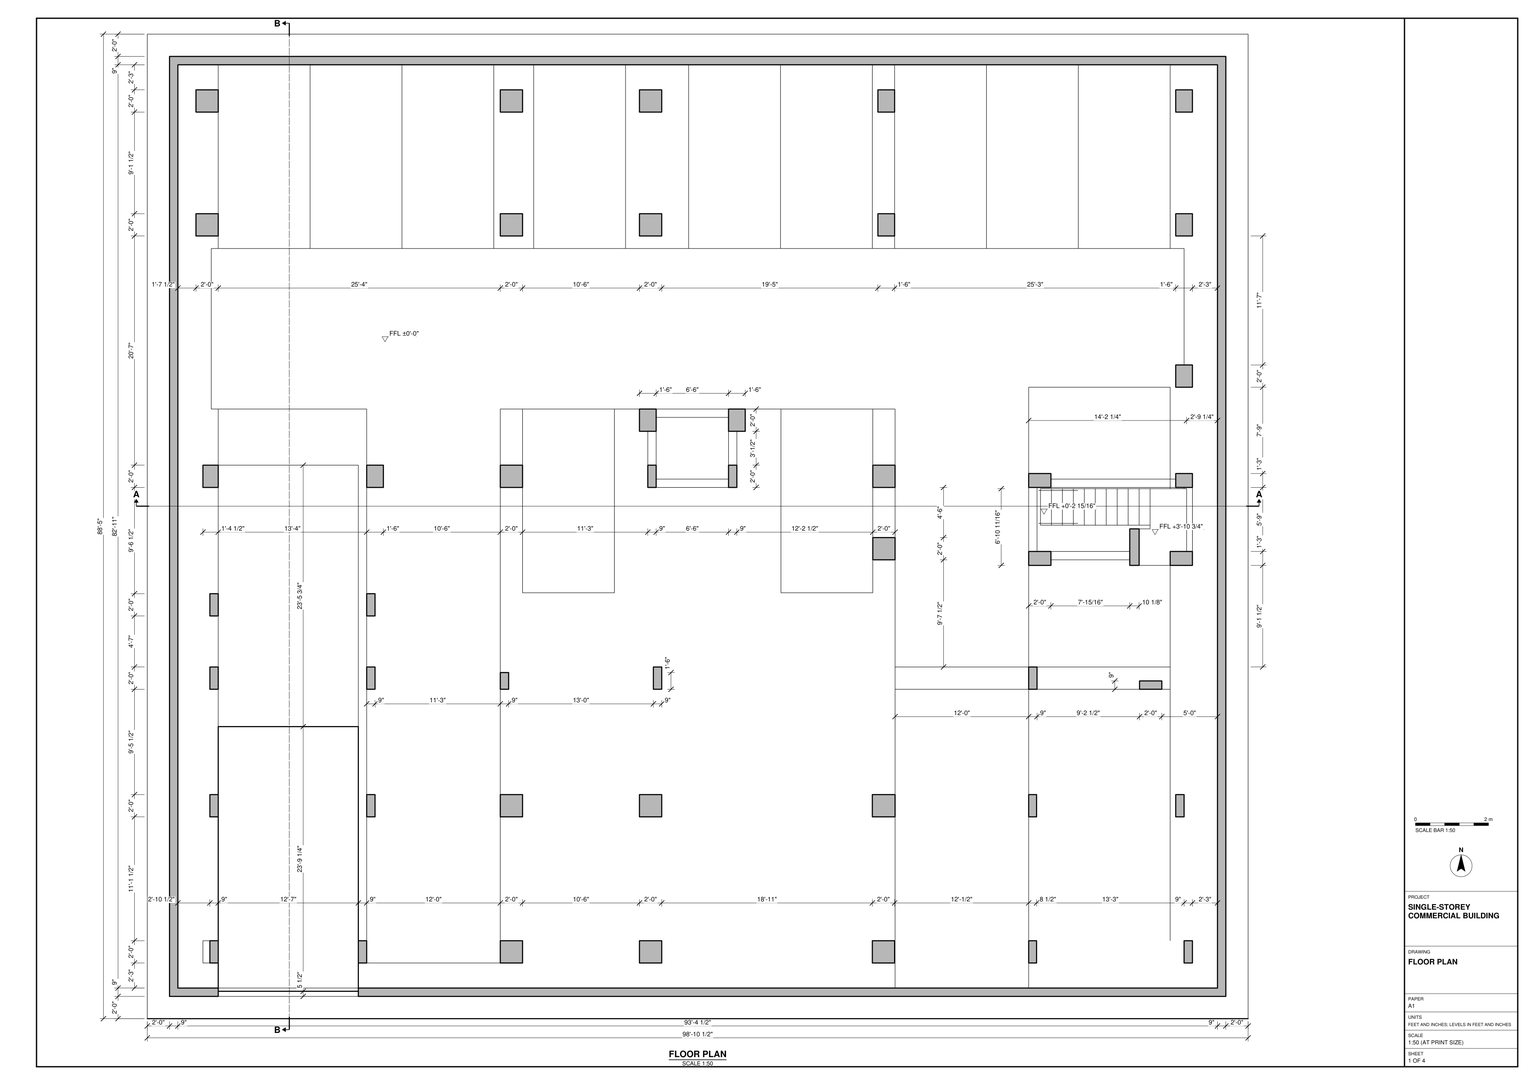
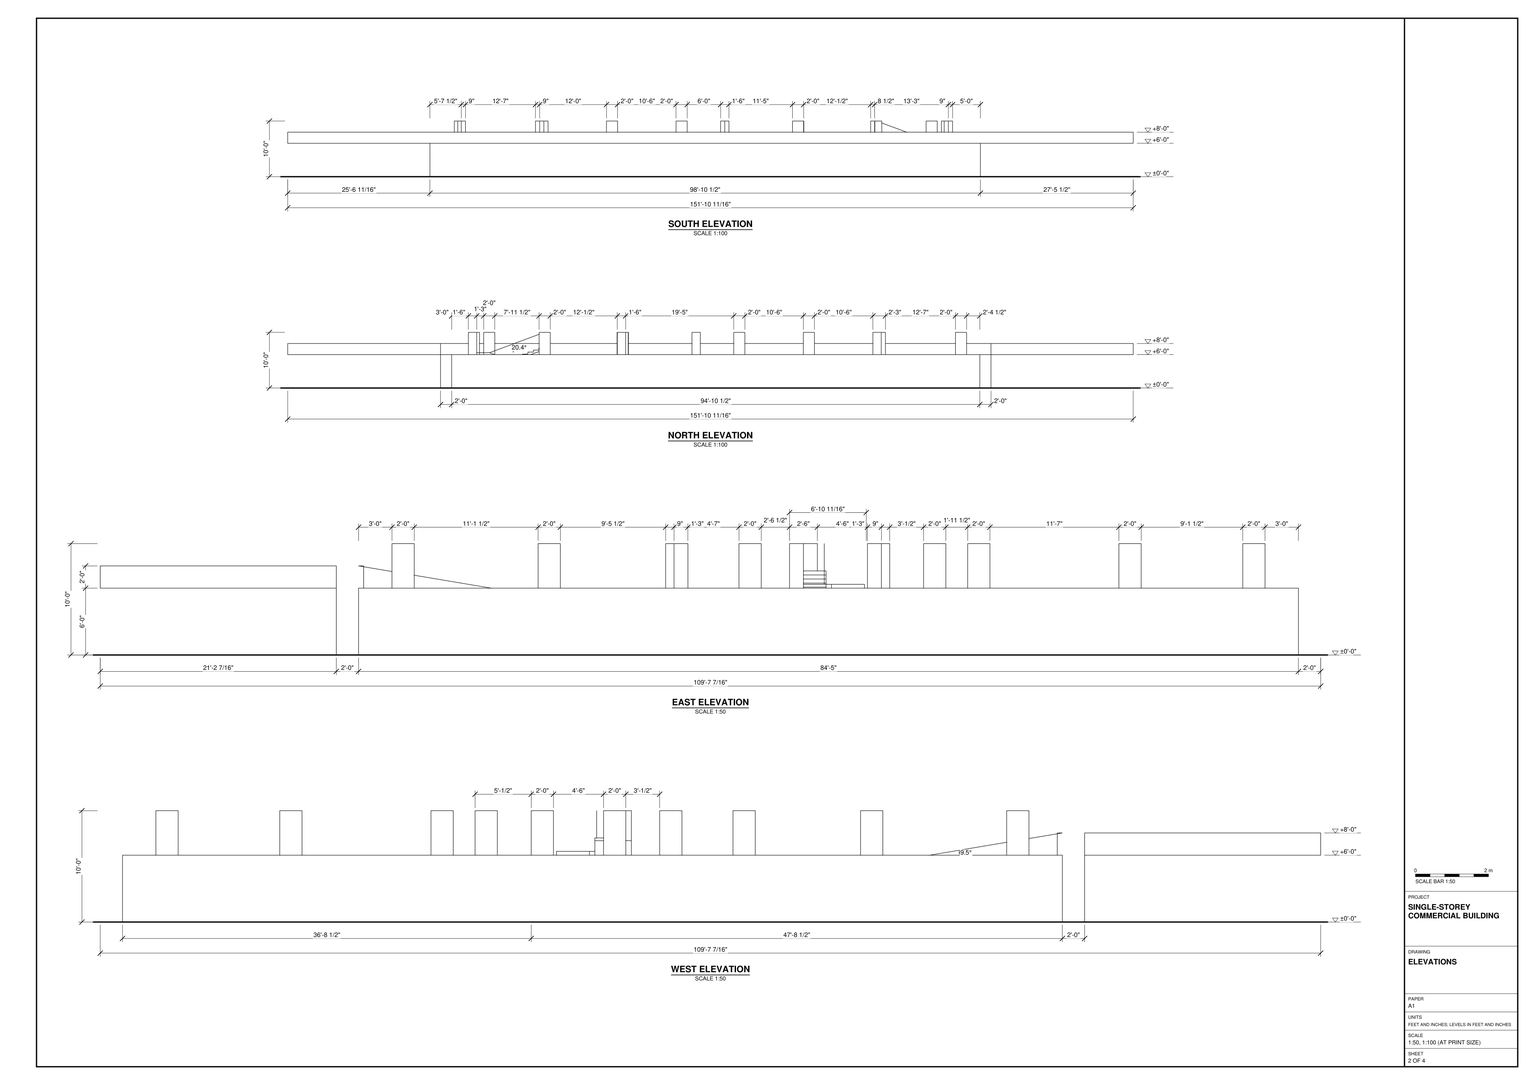
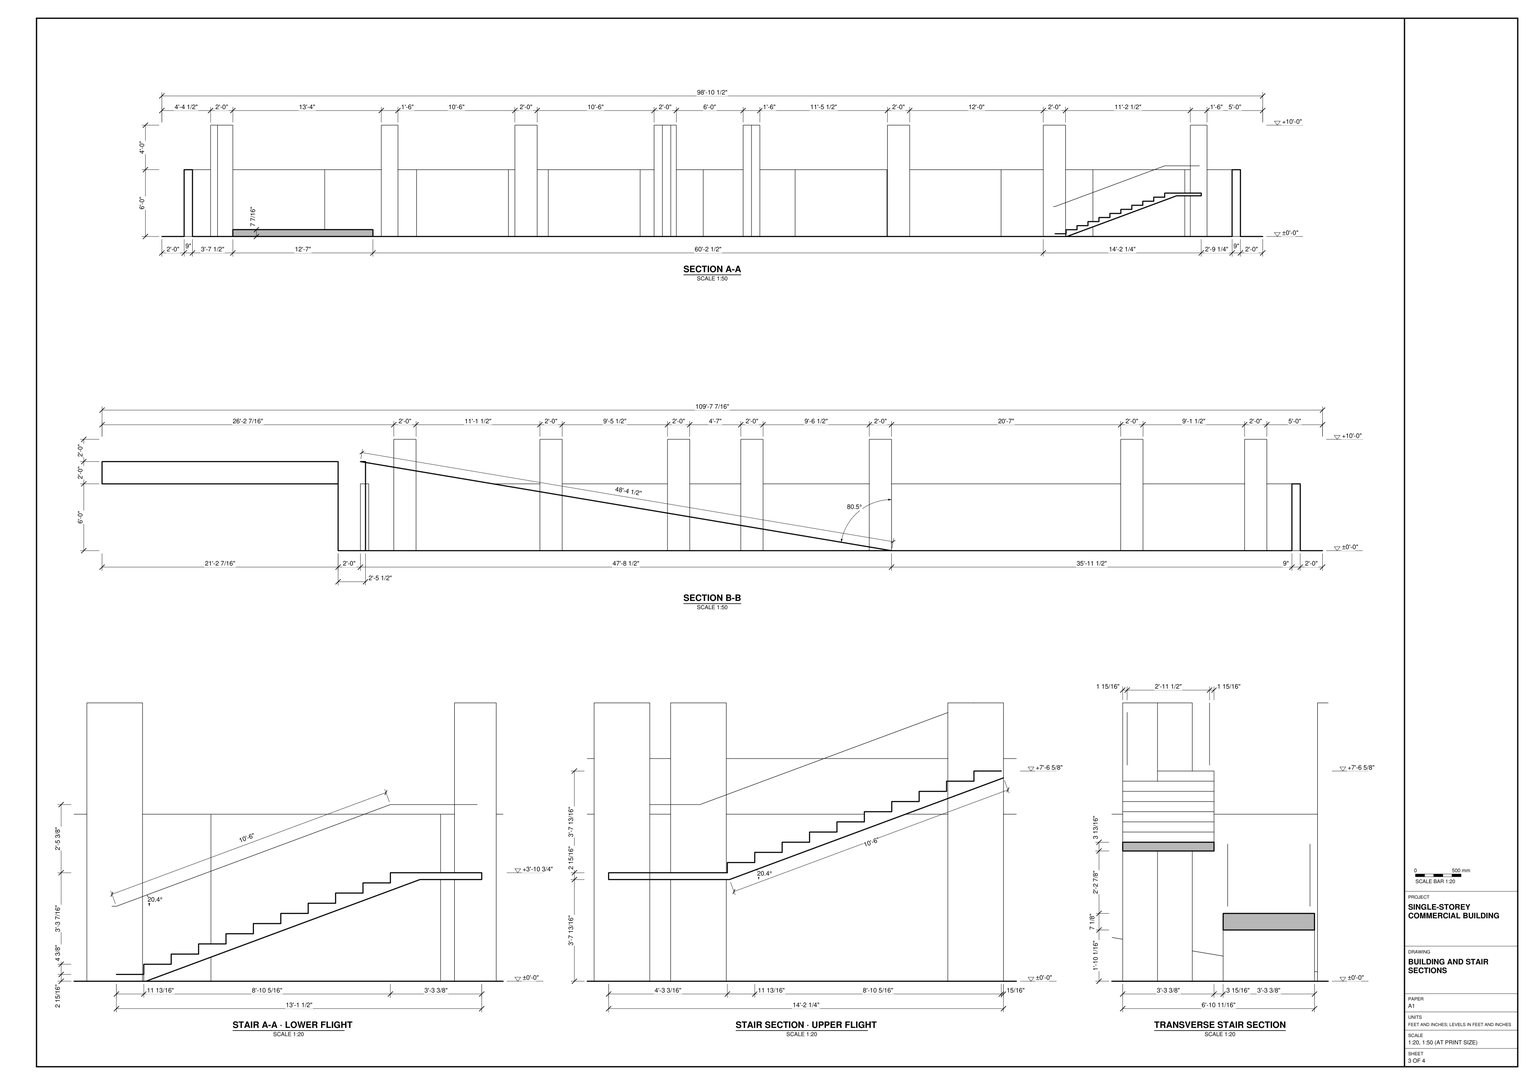
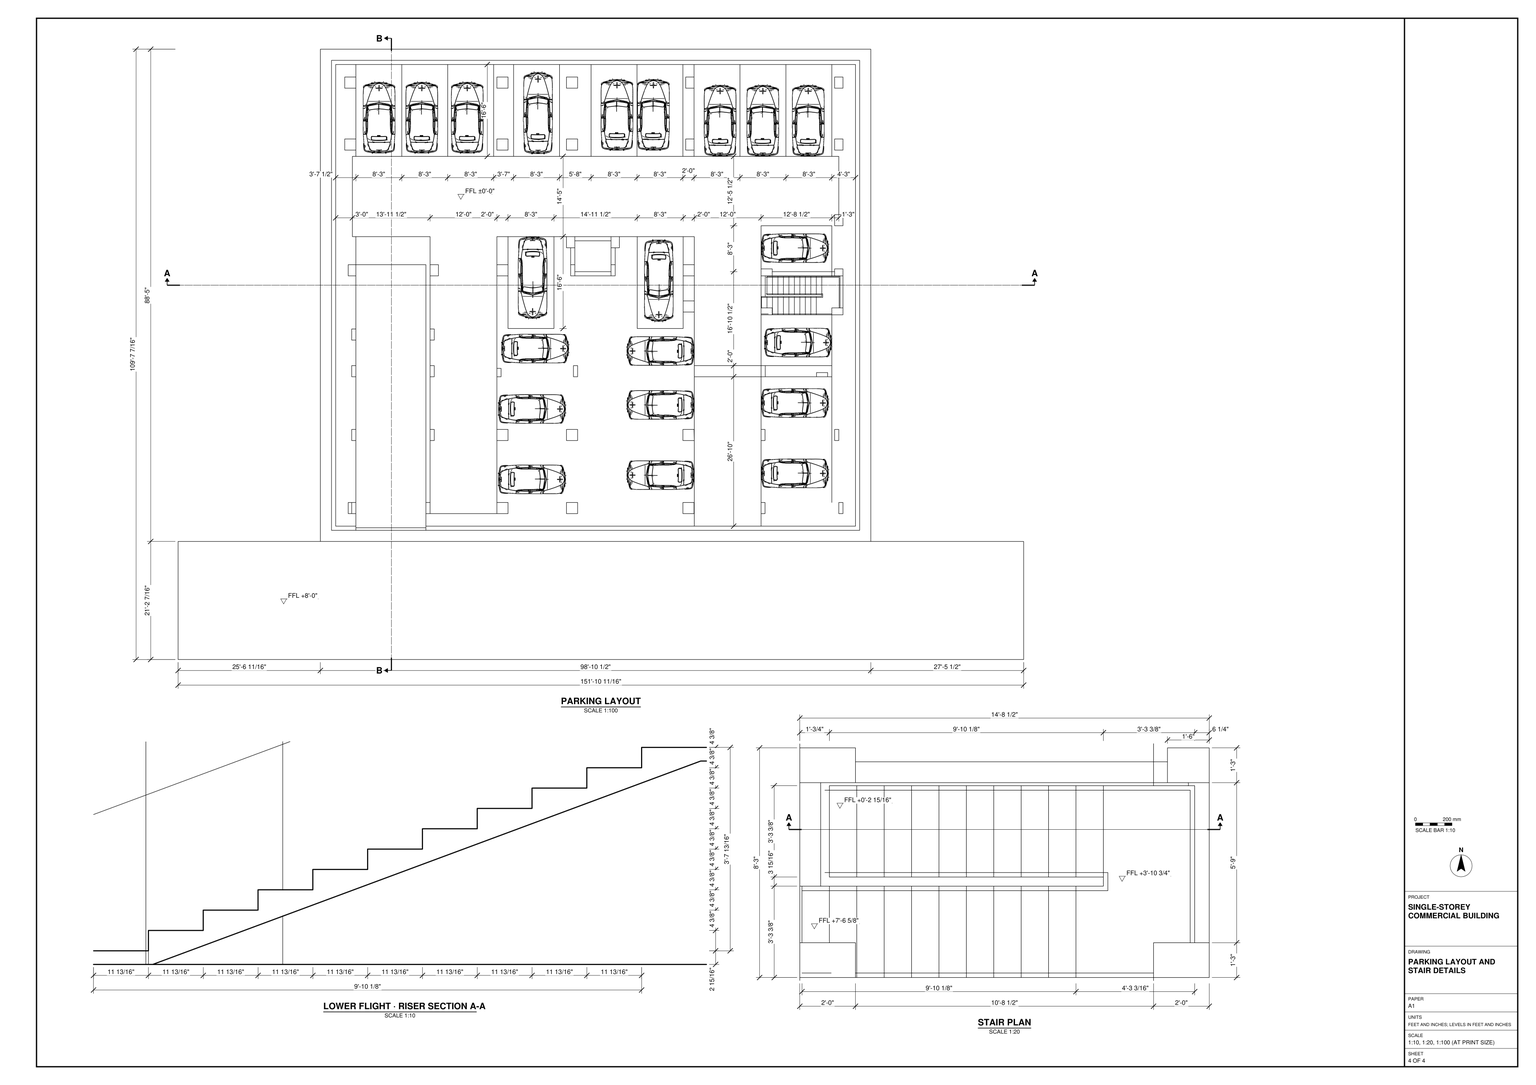
Build the single-storey commercial building in SketchUp from task_files/diagram_01.pdf. Work in feet and inches. Use ±0'-0" as the ground-floor level. The complete model measures 151'-10 11/16" east to west, 109'-7 7/16" north to south and 10'-0" high. These dimensions include the broad horizontal slab south of the enclosure; they are not the dimensions of the perimeter walls.

Lay out the ground slab, the 9" perimeter walls and the opening in the south wall from the floor plan. Place the rectangular posts using the individual bay dimensions; their footprints and spacing vary across the plan. Follow section B-B for the long ramp in the western bay, with its high end at the south wall and its low end at the ground floor. In the eastern bay, use the stair sections to model the lower flight, intermediate landing and returning upper flight. Match the slab and wall heights to the elevations, keeping the post tops visible above the walls.

Make walls, slabs, posts, ramp and stair separate groups or components, and use components for repeated parts. Keep each furniture or joinery piece shown separate. Any decor or loose items shown may be suitable library components. Save one SketchUp model as output_files/commercial_building_with_ramp_and_return_stair.skp.

# SketchUp Ruby script. Lengths in inches.
U = 1.inch
M = Sketchup.active_model
def pt(a) = Geom::Point3d.new(a.map { |v| v * U })
def face(e, loops, mat)
  f = e.add_face(loops[0].map { |a| pt(a) })
  loops[1..].each { |l| e.add_face(l.map { |a| pt(a) }).erase! }
  f.material = f.back_material = mat if mat
  f
end
# faces: each face lists its corners as indices into pts; further lists are holes
def faces(e, pts, list, mat = nil) = list.each { |f| face(e, (f[0].is_a?(Array) ? f : [f]).map { |l| l.map { |i| pts[i] } }, mat) }
# xy, xz, yz: faces in a plane at the given z, y or x. An outline is a flat list of corners, or four numbers for a rectangle; further outlines are holes
def ring(l) = l.size == 4 ? [[l[0], l[1]], [l[2], l[1]], [l[2], l[3]], [l[0], l[3]]] : l.each_slice(2).to_a
def flat(e, list, mat, &to3) = list.each { |f| face(e, (f[0].is_a?(Array) ? f : [f]).map { |l| ring(l).map { |u, v| to3.(u, v) } }, mat) }
def xy(e, z, list, mat = nil) = flat(e, list, mat) { |x, y| [x, y, z] }
def xz(e, y, list, mat = nil) = flat(e, list, mat) { |x, z| [x, y, z] }
def yz(e, x, list, mat = nil) = flat(e, list, mat) { |y, z| [x, y, z] }
def lines(e, pts, list) = list.each { |a, b| e.add_line(pt(pts[a]), pt(pts[b])) }
# prism: a flat outline (further loops are holes) pulled along v
def prism(e, loops, v, mat = nil)
  f = face(e, loops, mat); d = Geom::Vector3d.new(v.map { |x| x * U })
  f.pushpull(f.normal.samedirection?(d) ? d.length : -d.length)
end
def box(e, o, s, mat = nil) = prism(e, [[o, [o[0] + s[0], o[1], o[2]], [o[0] + s[0], o[1] + s[1], o[2]], [o[0], o[1] + s[1], o[2]]]], [0, 0, s[2]], mat)
def at(x, y, z, deg = 0) = Geom::Transformation.translation(pt([x, y, z])) * Geom::Transformation.rotation(ORIGIN, Z_AXIS, deg.degrees)
def axes(o, x, y, z) = Geom::Transformation.new([*x, 0, *y, 0, *z, 0, *pt(o).to_a, 1])
def part(name) = M.definitions.add(name)
# library, detail: a bought-in or finely detailed component or shape, given as its bounding box
def library(name, o, s) = part(name).tap { |d| box(d.entities, o, s) }
def detail(e, o, s) = box(e.add_group.entities, o, s)
def put(e, d, t, mat = nil) = e.add_instance(d, t).tap { |i| i.material = mat if mat }
def group(e, t, mat = nil) = e.add_group.tap { |g| g.transformation = t; g.material = mat if mat }.entities
root = M.entities
c1 = library("1948+packard",[-10.22,-85.54,-0.68],[196.68,537.21,187.22])
c2 = part("Access ramp")
xy(c2.entities,0,[[0,2.37,92.45,245.94]])
xy(c2.entities,121.68,[[0,0,92.45,2.37]])
xz(c2.entities,2.37,[[0,0,92.45,121.68]])
yz(c2.entities,0,[[2.37,0,2.37,121.68,0,121.68,2.37,120.51,245.94,0]])
yz(c2.entities,92.45,[[2.37,0,245.94,0,2.37,120.51,0,121.68,2.37,121.68]])
p = [[92.45,245.94,0],[0,245.94,0],[0,2.37,120.51],[0,0,121.68],[92.45,0,121.68],[92.45,2.37,120.51]]
faces(c2.entities,p,[[0,1,2,3,4,5]])
c3 = part("Group1\#1")
box(c3.entities,[611.99,1440.83,0],[24,24,120])
c4 = part("Group2\#1")
box(c4.entities,[939.99,1440.83,0],[24,24,120])
c5 = part("Group3\#1")
box(c5.entities,[939.99,681.33,0],[24,24,120])
c6 = part("Group4\#1")
box(c6.entities,[1089.99,681.33,0],[24,24,120])
c7 = part("Group5\#1")
box(c7.entities,[1340.99,681.33,0],[24.5,24,120])
c8 = part("Group7\#1")
box(c8.entities,[939.99,818.83,0],[9,18,120])
c9 = part("Group9\#1")
box(c9.entities,[1667.99,1307.33,0],[18,24,120])
c10 = part("Group10\#1")
box(c10.entities,[1667.99,1440.83,0],[18,24,120])
c11 = part("Group11\#1")
box(c11.entities,[1346.99,1440.83,0],[18,24,120])
c12 = part("Group12\#1")
box(c12.entities,[1346.99,1307.33,0],[18,24,120])
c13 = part("Group13\#1")
box(c13.entities,[1667.99,1144.33,0],[18,24,120])
c14 = part("Group14\#1")
box(c14.entities,[1676.99,523.83,0],[9,24,120])
c15 = part("Group15\#1")
box(c15.entities,[1667.99,681.33,0],[9,24,120])
c16 = part("Group16\#1")
box(c16.entities,[1509.49,681.33,0],[8.5,24,120])
c17 = part("Group18\#1")
box(c17.entities,[1509.49,523.83,0],[8.5,24,120])
c18 = part("Group17\#1")
box(c18.entities,[1104.99,818.83,0],[9,24,120])
c19 = part("Group19\#1")
box(c19.entities,[786.99,523.83,0],[9,24,120])
c20 = part("Group20\#1")
box(c20.entities,[626.99,523.83,0],[9,24,120])
c21 = part("Group20\#2")
box(c21.entities,[626.99,681.33,0],[9,24,120])
c22 = part("Group21\#1")
box(c22.entities,[626.99,818.83,0],[9,24,120])
c23 = part("Group22\#1")
box(c23.entities,[626.99,897.83,0],[9,24,120])
c24 = part("Group23\#1")
box(c24.entities,[619.49,1036.33,0],[16.5,24,120])
c25 = part("Group24\#1")
box(c25.entities,[795.99,1036.33,0],[18,24,120])
c26 = part("Group25\#1")
box(c26.entities,[939.99,1036.33,0],[24,24,120])
c27 = part("Group26\#1")
box(c27.entities,[1341.49,1036.33,0],[24,24,120])
c28 = part("Group28\#1")
box(c28.entities,[1509.49,1036.33,0],[24,15,120])
c29 = part("Group29\#1")
box(c29.entities,[1667.99,1036.33,0],[18,15,120])
c30 = part("Group30\#1")
box(c30.entities,[1509.49,952.33,0],[24,15,120])
c31 = part("Group31\#1")
box(c31.entities,[1661.99,952.33,0],[24,15,120])
c32 = part("Group33\#1")
p = [[1520.43,876.89,0],[1520.43,878.83,0],[1520.43,996.95,58.75],[1520.43,1034.39,58.75],[1599.24,1034.39,58.75],[1599.24,996.95,58.75],
  [1599.24,878.83,117.5],[1599.24,867.02,117.5],[1555.93,876.89,0],[1555.93,878.83,0],[1555.93,996.95,58.75],[1555.93,998.89,58.75],
  [1563.74,998.89,58.75],[1563.74,996.95,58.75],[1563.74,878.83,117.5],[1563.74,867.02,117.5]]
lines(c32.entities,p,[[0,1],[1,2],[2,3],[3,4],[4,5],[5,6],[6,7],[8,9],[9,10],[10,11],[11,12],[12,13],
  [13,14],[14,15]])
c33 = part("Group32\#1")
xy(c33.entities,-3.9375,[[1518.49,890.64,1557.87,891.57]])
xy(c33.entities,0,[[1518.49,878.83,1557.87,890.64]])
xy(c33.entities,5.875,[[1518.49,890.64,1557.87,902.45]])
xy(c33.entities,11.75,[[1518.49,902.45,1557.87,914.27]])
xy(c33.entities,17.625,[[1518.49,914.27,1557.87,926.08]])
xy(c33.entities,23.5,[[1518.49,926.08,1557.87,937.89]])
xy(c33.entities,29.375,[[1518.49,937.89,1557.87,949.7]])
xy(c33.entities,35.25,[[1518.49,949.7,1557.87,961.52]])
xy(c33.entities,41.125,[[1518.49,961.52,1557.87,973.33]])
xy(c33.entities,47,[[1518.49,973.33,1557.87,985.14]])
xy(c33.entities,52.875,[[1518.49,985.14,1557.87,996.95]])
xy(c33.entities,54.8125,[[1561.81,984.22,1561.81,996.95,1557.87,996.95,1557.87,1009.69,1518.49,1009.69,1518.49,1036.33,1601.18,1036.33,1601.18,984.22]])
xy(c33.entities,58.75,[[1561.81,985.14,1601.18,985.14,1601.18,1036.33,1518.49,1036.33,1518.49,996.95,1561.81,996.95]])
xy(c33.entities,64.625,[[1561.81,973.33,1601.18,985.14]])
xy(c33.entities,70.5,[[1561.81,961.52,1601.18,973.33]])
xy(c33.entities,76.375,[[1561.81,949.7,1601.18,961.52]])
xy(c33.entities,82.25,[[1561.81,937.89,1601.18,949.7]])
xy(c33.entities,88.125,[[1561.81,926.08,1601.18,937.89]])
xy(c33.entities,94,[[1561.81,914.27,1601.18,926.08]])
xy(c33.entities,99.875,[[1561.81,902.45,1601.18,914.27]])
xy(c33.entities,105.75,[[1561.81,890.64,1601.18,902.45]])
xy(c33.entities,111.625,[[1561.81,878.83,1601.18,890.64]])
xy(c33.entities,117.5,[[1561.81,867.02,1601.18,878.83]])
xz(c33.entities,878.83,[[1561.81,111.625,1601.18,117.5]])
xz(c33.entities,890.64,[[1518.49,0,1557.87,5.875],[1561.81,105.75,1601.18,111.625]])
xz(c33.entities,902.45,[[1518.49,5.875,1557.87,11.75],[1561.81,99.875,1601.18,105.75]])
xz(c33.entities,914.27,[[1518.49,11.75,1557.87,17.625],[1561.81,94,1601.18,99.875]])
xz(c33.entities,926.08,[[1518.49,17.625,1557.87,23.5],[1561.81,88.125,1601.18,94]])
xz(c33.entities,937.89,[[1518.49,23.5,1557.87,29.375],[1561.81,82.25,1601.18,88.125]])
xz(c33.entities,949.7,[[1518.49,29.375,1557.87,35.25],[1561.81,76.375,1601.18,82.25]])
xz(c33.entities,961.52,[[1518.49,35.25,1557.87,41.125],[1561.81,70.5,1601.18,76.375]])
xz(c33.entities,973.33,[[1518.49,41.125,1557.87,47],[1561.81,64.625,1601.18,70.5]])
xz(c33.entities,985.14,[[1518.49,47,1557.87,52.875],[1561.81,58.75,1601.18,64.625]])
xz(c33.entities,996.95,[[1518.49,52.875,1557.87,58.75],[1557.87,54.8125,1561.81,58.75]])
xz(c33.entities,1036.33,[[1518.49,54.8125,1601.18,58.75]])
yz(c33.entities,1518.49,[[890.64,-3.9375,890.64,5.875,902.45,5.875,902.45,11.75,914.27,11.75,914.27,17.625,926.08,17.625,926.08,23.5,937.89,23.5,937.89,29.375,949.7,29.375,949.7,35.25,961.52,35.25,961.52,41.125,973.33,41.125,973.33,47,985.14,47,985.14,52.875,996.95,52.875,996.95,58.75,1036.33,58.75,1036.33,54.8125,1009.69,54.8125,891.57,-3.9375]])
yz(c33.entities,1557.87,[[890.64,-3.9375,891.57,-3.9375,1009.69,54.8125,996.95,54.8125,996.95,52.875,985.14,52.875,985.14,47,973.33,47,973.33,41.125,961.52,41.125,961.52,35.25,949.7,35.25,949.7,29.375,937.89,29.375,937.89,23.5,926.08,23.5,926.08,17.625,914.27,17.625,914.27,11.75,902.45,11.75,902.45,5.875,890.64,5.875]])
yz(c33.entities,1561.81,[[984.22,54.8125,866.09,113.5625,867.02,113.5625,867.02,117.5,878.83,117.5,878.83,111.625,890.64,111.625,890.64,105.75,902.45,105.75,902.45,99.875,914.27,99.875,914.27,94,926.08,94,926.08,88.125,937.89,88.125,937.89,82.25,949.7,82.25,949.7,76.375,961.52,76.375,961.52,70.5,973.33,70.5,973.33,64.625,985.14,64.625,985.14,58.75,996.95,58.75,996.95,54.8125]])
yz(c33.entities,1601.18,[[984.22,54.8125,1036.33,54.8125,1036.33,58.75,985.14,58.75,985.14,64.625,973.33,64.625,973.33,70.5,961.52,70.5,961.52,76.375,949.7,76.375,949.7,82.25,937.89,82.25,937.89,88.125,926.08,88.125,926.08,94,914.27,94,914.27,99.875,902.45,99.875,902.45,105.75,890.64,105.75,890.64,111.625,878.83,111.625,878.83,117.5,867.02,117.5,867.02,113.5625,866.09,113.5625]])
p = [[1518.49,891.57,-3.9375],[1518.49,1009.69,54.8125],[1557.87,1009.69,54.8125],[1557.87,891.57,-3.9375],[1601.18,984.22,54.8125],[1601.18,866.09,113.5625],
  [1561.81,866.09,113.5625],[1561.81,984.22,54.8125]]
faces(c33.entities,p,[[0,1,2,3],[4,5,6,7]])
put(c33.entities,c32,at(0,0,39.375))
c34 = part("Group34\#1")
box(c34.entities,[1089.99,1096.83,0],[18,24,120])
xy(root,0,[[[306.6875,254.4375,1493.1875,1315.4375],[330.6875,278.4375,1469.1875,1291.4375]],[383.1875,278.4375,534.1875,287.4375],[[339.6875,287.4375,534.1875,287.4375,534.1875,338.4375,543.1875,338.4375,543.1875,911.4375,375.6875,911.4375,375.6875,1084.4375,383.1875,1084.4375,383.1875,1097.9375,359.1875,1097.9375,359.1875,1121.9375,383.1875,1121.9375,383.1875,1231.4375,359.1875,1231.4375,359.1875,1255.4375,383.1875,1255.4375,383.1875,1282.4375,339.6875,1282.4375],[366.6875,826.9375,383.1875,850.9375],[374.1875,471.9375,383.1875,495.9375],[366.6875,314.4375,375.6875,338.4375]],[[1256.6875,287.4375,1460.1875,287.4375,1460.1875,1282.4375,1409.1875,1282.4375,1409.1875,1084.4375,1424.1875,1084.4375,1424.1875,958.9375,1433.1875,958.9375,1433.1875,934.9375,1415.1875,934.9375,1415.1875,958.9375,1424.1875,958.9375,1424.1875,1084.4375,375.6875,1084.4375,375.6875,911.4375,543.1875,911.4375,543.1875,850.9375,561.1875,850.9375,561.1875,826.9375,543.1875,826.9375,543.1875,314.4375,687.1875,314.4375,687.1875,911.4375,1112.6875,911.4375,1112.6875,633.4375,1409.1875,633.4375,1409.1875,609.4375,1256.6875,609.4375],[1280.6875,835.9375,1280.6875,841.9375,1256.6875,841.9375,1256.6875,934.9375,1409.1875,934.9375,1409.1875,835.9375],[1415.1875,1097.9375,1433.1875,1121.9375],[1415.1875,1231.4375,1433.1875,1255.4375],[1424.1875,314.4375,1433.1875,338.4375]],[[534.1875,287.4375,1112.6875,287.4375,1112.6875,826.9375,1088.6875,826.9375,1088.6875,713.4375,989.6875,713.4375,989.6875,911.4375,951.1875,911.4375,951.1875,887.4375,933.1875,887.4375,933.1875,902.4375,855.1875,902.4375,855.1875,887.4375,837.1875,887.4375,837.1875,911.4375,810.1875,911.4375,810.1875,713.4375,711.1875,713.4375,711.1875,826.9375,687.1875,826.9375,687.1875,627.4375,696.1875,627.4375,696.1875,609.4375,687.1875,609.4375,687.1875,495.9375,711.1875,495.9375,711.1875,471.9375,687.1875,471.9375,687.1875,338.4375,711.1875,338.4375,711.1875,314.4375,534.1875,314.4375],[837.1875,471.9375,861.1875,495.9375],[837.1875,314.4375,861.1875,338.4375],[852.1875,609.4375,861.1875,627.4375]],
  [1112.6875,287.4375,1256.6875,609.4375],[366.6875,314.4375,375.6875,338.4375],[534.1875,314.4375,543.1875,338.4375],[687.1875,314.4375,711.1875,338.4375],[837.1875,314.4375,861.1875,338.4375],
  [1088.1875,314.4375,1112.6875,314.4375,1112.1875,338.4375,1088.1875,338.4375],[1424.1875,314.4375,1433.1875,338.4375],[374.1875,471.9375,383.1875,495.9375],[687.1875,471.9375,711.1875,495.9375],[837.1875,471.9375,861.1875,495.9375],
  [1088.1875,471.9375,1112.6875,471.9375,1112.1875,495.9375,1088.1875,495.9375],[687.1875,609.4375,696.1875,627.4375],[852.1875,609.4375,861.1875,627.4375],[1112.6875,609.4375,1112.6875,633.4375,1409.1875,633.4375,1409.1875,748.9375,1280.6875,748.9375,1280.6875,742.9375,1256.6875,742.9375,1256.6875,826.9375,1265.6875,826.9375,1265.6875,757.9375,1280.6875,748.9375,1280.6875,742.9375,1256.6875,742.9375,1256.6875,609.4375],[1112.6875,609.4375,1256.6875,633.4375],
  [1256.6875,609.4375,1409.1875,633.4375],[1256.6875,633.4375,1409.1875,633.4375,1409.1875,748.9375,1280.6875,748.9375,1280.6875,742.9375,1256.6875,742.9375],[711.1875,713.4375,810.1875,911.4375],[989.6875,713.4375,1088.6875,911.4375],[1280.6875,748.9375,1280.6875,757.9375,1409.1875,757.9375,1409.1875,826.9375,1265.6875,826.9375,1265.6875,757.9375],
  [1280.6875,748.9375,1409.1875,757.9375],[366.6875,826.9375,374.1875,850.9375],[374.1875,826.9375,383.1875,850.9375],[543.1875,826.9375,561.1875,850.9375],[687.1875,826.9375,711.1875,850.9375],
  [1088.6875,826.9375,1112.6875,850.9375],[1256.6875,826.9375,1280.6875,841.9375],[1280.6875,826.9375,1409.1875,835.9375],[1280.6875,835.9375,1409.1875,835.9375,1409.1875,934.9375,1256.6875,934.9375,1256.6875,841.9375,1280.6875,841.9375],[687.1875,850.9375,711.1875,911.4375],
  [1088.6875,850.9375,1112.6875,911.4375],[837.1875,887.4375,855.1875,911.4375],[933.1875,887.4375,951.1875,911.4375],[855.1875,902.4375,933.1875,911.4375],[1415.1875,934.9375,1433.1875,958.9375],
  [383.1875,1084.4375,482.1875,1282.4375],[482.1875,1084.4375,581.1875,1282.4375],[581.1875,1084.4375,680.1875,1282.4375],[[680.1875,1084.4375,723.1875,1282.4375],[687.1875,1231.4375,711.1875,1255.4375],[687.1875,1097.9375,711.1875,1121.9375]],[723.1875,1084.4375,822.1875,1282.4375],
  [[822.1875,1084.4375,890.1875,1282.4375],[837.1875,1231.4375,861.1875,1255.4375],[837.1875,1097.9375,861.1875,1121.9375]],[890.1875,1084.4375,989.1875,1282.4375],[989.1875,1084.4375,1088.1875,1282.4375],[1088.1875,1084.4375,1112.1875,1084.4375,1112.1875,1097.9375,1094.1875,1097.9375,1094.1875,1121.9375,1112.1875,1121.9375,1112.1875,1231.4375,1094.1875,1231.4375,1094.1875,1255.4375,1112.1875,1255.4375,1112.1875,1282.4375,1088.1875,1282.4375],[1112.1875,1084.4375,1211.1875,1282.4375],
  [1211.1875,1084.4375,1310.1875,1282.4375],[1310.1875,1084.4375,1409.1875,1282.4375],[359.1875,1097.9375,383.1875,1121.9375],[687.1875,1097.9375,711.1875,1121.9375],[837.1875,1097.9375,861.1875,1121.9375],
  [1094.1875,1097.9375,1112.1875,1121.9375],[1415.1875,1097.9375,1433.1875,1121.9375],[359.1875,1231.4375,383.1875,1255.4375],[687.1875,1231.4375,711.1875,1255.4375],[837.1875,1231.4375,861.1875,1255.4375],
  [1094.1875,1231.4375,1112.1875,1255.4375],[1415.1875,1231.4375,1433.1875,1255.4375]])
xy(root,72,[[0,0,1822.6875,254.4375],[330.6875,278.4375,383.1875,278.4375,383.1875,287.4375,339.6875,287.4375,339.6875,1282.4375,1460.1875,1282.4375,1460.1875,287.4375,534.1875,287.4375,534.1875,278.4375,1469.1875,278.4375,1469.1875,1291.4375,330.6875,1291.4375]])
xy(root,96,[[0,0,1822.6875,254.4375]])
xz(root,0,[[0,72,1822.6875,96]])
xz(root,254.4375,[[306.6875,0,1493.1875,72],[0,72,306.6875,96],[306.6875,72,1493.1875,96],[1493.1875,72,1822.6875,96]])
xz(root,278.4375,[[330.6875,0,383.1875,72],[534.1875,0,1469.1875,72]])
xz(root,287.4375,[[339.6875,0,383.1875,72],[534.1875,0,543.1875,72],[543.1875,0,687.1875,72],[687.1875,0,1112.6875,72],[1112.6875,0,1256.6875,72],
  [1256.6875,0,1460.1875,72]])
xz(root,1282.4375,[[339.6875,0,383.1875,72],[383.1875,0,482.1875,72],[482.1875,0,581.1875,72],[581.1875,0,680.1875,72],[680.1875,0,723.1875,72],
  [723.1875,0,822.1875,72],[822.1875,0,890.1875,72],[890.1875,0,989.1875,72],[989.1875,0,1088.1875,72],[1088.1875,0,1112.1875,72],
  [1112.1875,0,1211.1875,72],[1211.1875,0,1310.1875,72],[1310.1875,0,1409.1875,72],[1409.1875,0,1460.1875,72]])
xz(root,1291.4375,[[330.6875,0,1469.1875,72]])
yz(root,0,[[0,72,254.4375,96]])
yz(root,330.6875,[[278.4375,0,1291.4375,72]])
yz(root,339.6875,[[287.4375,0,1282.4375,72]])
yz(root,383.1875,[[278.4375,0,287.4375,72]])
yz(root,534.1875,[[278.4375,0,287.4375,72]])
yz(root,1460.1875,[[287.4375,0,1282.4375,72]])
yz(root,1469.1875,[[278.4375,0,1291.4375,72]])
yz(root,1822.6875,[[0,72,254.4375,96]])
p = [[1409.1875,338.4375,0],[1409.1875,609.4375,0],[383.1875,911.4375,0],[383.1875,850.9375,0],[383.1875,471.9375,0],[383.1875,330.9375,0],
  [383.1875,826.9375,0],[383.1875,495.9375,0],[1433.1875,742.9375,0],[1415.1875,742.9375,0],[1409.1875,742.9375,0],[1409.1875,826.9375,0],
  [1415.1875,826.9375,0],[1433.1875,757.9375,0],[1433.1875,826.9375,0],[1424.1875,826.9375,0],[1424.1875,757.9375,0],[1415.1875,835.9375,0],
  [1409.1875,835.9375,0],[933.1875,887.4375,0],[933.1875,835.9375,0],[855.1875,850.9375,0],[855.1875,887.4375,0],[855.1875,835.9375,0],
  [933.1875,826.9375,0],[855.1875,826.9375,0],[846.1875,850.9375,0],[846.1875,887.4375,0],[942.1875,850.9375,0],[942.1875,887.4375,0],
  [383.1875,314.4375,0],[383.1875,287.4375,0]]
lines(root,p,[[0,1],[2,3],[4,5],[6,7],[8,9],[9,10],[11,12],[13,14],[15,16],[17,18],[19,20],[21,22],
  [23,20],[20,24],[24,25],[26,27],[28,29],[30,31]])
put(root,c1,axes([804.1,1238.39,0.34],[-0.32,0,0],[0,-0.33,0],[0,0,0.5]))
put(root,c1,axes([1389.63,1214.11,0.34],[-0.35482,0,0],[0,-0.2871,0],[0,0,0.5]))
put(root,c1,axes([1291.7,1214.11,0.34],[-0.35482,0,0],[0,-0.2871,0],[0,0,0.5]))
put(root,c1,axes([1291.7,1214.11,0.34],[-0.35482,0,0],[0,-0.2871,0],[0,0,0.5]))
put(root,c1,axes([1199.63,1214.11,0.34],[-0.35482,0,0],[0,-0.2871,0],[0,0,0.5]))
put(root,c1,axes([654.54,1220.54,0.34],[-0.35482,0,0],[0,-0.2871,0],[0,0,0.5]))
put(root,c1,axes([464.54,1220.54,0.34],[-0.35482,0,0],[0,-0.2871,0],[0,0,0.5]))
put(root,c1,axes([556.6,1220.54,0.34],[-0.35482,0,0],[0,-0.2871,0],[0,0,0.5]))
put(root,c1,axes([1055.85,1226.66,0.34],[-0.35482,0,0],[0,-0.2871,0],[0,0,0.5]))
put(root,c1,axes([977.29,1226.66,0.34],[-0.35482,0,0],[0,-0.2871,0],[0,0,0.5]))
put(root,c1,axes([1008.02,755.94,0.34],[0.32,0,0],[0,0.33,0],[0,0,0.5]))
put(root,c1,axes([735.97,762.38,0.34],[0.32,0,0],[0,0.33,0],[0,0,0.5]))
put(root,c1,axes([1379.46,858.39,0.34],[0,0.32,0],[-0.27181,0,0],[0,0,0.5]))
put(root,c1,axes([1386.29,654.85,0.34],[0,0.32,0],[-0.27181,0,0],[0,0,0.5]))
put(root,c1,axes([1379.46,524.65,0.34],[0,0.32,0],[-0.27181,0,0],[0,0,0.5]))
put(root,c1,axes([1379.46,372.93,0.34],[0,0.32,0],[-0.27181,0,0],[0,0,0.5]))
put(root,c1,axes([819.57,641.96,0.34],[0,0.32,0],[-0.27181,0,0],[0,0,0.5]))
put(root,c1,axes([812.74,360.04,0.34],[0,0.32,0],[-0.27181,0,0],[0,0,0.5]))
put(root,c1,axes([812.74,511.76,0.34],[0,0.32,0],[-0.27181,0,0],[0,0,0.5]))
put(root,c1,axes([989.92,693.1,0.34],[0,-0.32,0],[0.27181,0,0],[0,0,0.5]))
put(root,c1,axes([989.92,576.96,0.34],[0,-0.32,0],[0.27181,0,0],[0,0,0.5]))
put(root,c1,axes([989.92,425.57,0.34],[0,-0.32,0],[0.27181,0,0],[0,0,0.5]))
put(root,c2,axes([383.1875,278.4375,0],[1.6334,0,0],[0,2.3278,0],[0,0,0.78895]))
put(root,c3,at(-252.81,-209.39,0))
put(root,c4,at(-252.81,-209.39,0))
put(root,c4,at(-252.81,-342.89,0))
put(root,c4,at(-102.81,-342.89,0))
put(root,c4,at(-102.81,-209.39,0))
put(root,c4,at(-580.81,-342.89,0))
put(root,c4,at(-252.81,-1126.39,0))
put(root,c4,at(-102.81,-1126.39,0))
put(root,c4,at(148.19,-1126.39,0))
put(root,c5,at(-252.81,-209.39,0))
put(root,c6,at(-252.81,-209.39,0))
put(root,c7,at(-252.81,-209.39,0))
put(root,c8,at(-252.81,-209.39,0))
put(root,c9,at(-252.81,-209.39,0))
put(root,c10,at(-252.81,-209.39,0))
put(root,c11,at(-252.81,-209.39,0))
put(root,c12,at(-252.81,-209.39,0))
put(root,c13,at(-252.81,-209.39,0))
put(root,c14,at(-252.81,-209.39,0))
put(root,c15,at(-252.81,-209.39,0))
put(root,c16,at(-252.81,-209.39,0))
put(root,c17,at(-252.81,-209.39,0))
put(root,c18,at(-252.81,-209.39,0))
put(root,c19,at(-252.81,-209.39,0))
put(root,c20,at(-252.81,-209.39,0))
put(root,c21,at(-252.81,-209.39,0))
put(root,c22,at(-252.81,-209.39,0))
put(root,c23,at(-252.81,-209.39,0))
put(root,c24,at(-252.81,-209.39,0))
put(root,c25,at(-252.81,-209.39,0))
put(root,c26,at(-252.81,-209.39,0))
put(root,c27,at(-252.81,-209.39,0))
put(root,c28,at(-252.81,-209.39,0))
put(root,c29,at(-252.81,-209.39,0))
put(root,c30,at(-252.81,-209.39,0))
put(root,c31,at(-252.81,-209.39,0))
put(root,c33,axes([390.6,2344.12,2.9375],[0,-1,0],[1,0,0],[0,0,0.74621]))
put(root,c23,at(-83.81,-209.39,0))
put(root,c23,at(-83.81,-288.39,0))
put(root,c23,at(-83.81,-425.89,0))
put(root,c27,at(-252.81,-287.39,0))
put(root,c34,at(-252.81,-209.39,0))
put(root,c34,at(-156.81,-209.39,0))
put(root,c23,at(219.19,-70.89,0))
put(root,c23,at(306.19,-70.89,0))
put(root,c18,at(151.69,-209.39,0))
put(root,c18,at(2219.02,-495.56,0,90))
